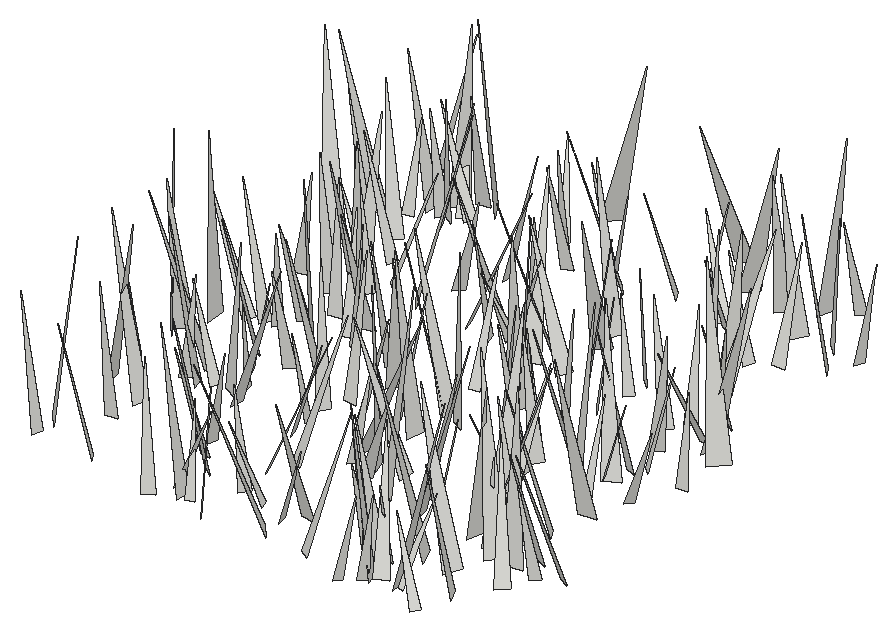
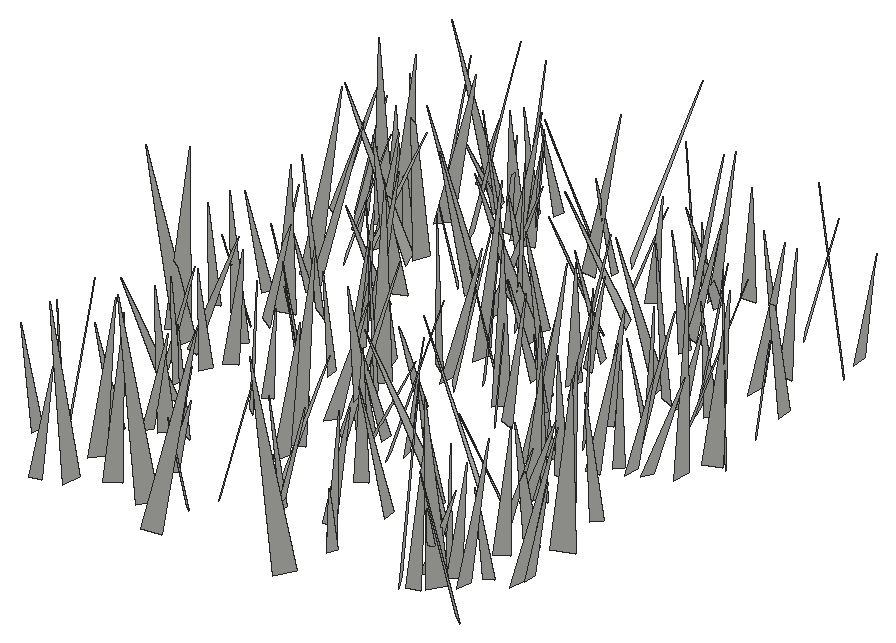
# SketchUp Ruby script. Lengths in inches.
U = 1.inch
M = Sketchup.active_model
def pt(a) = Geom::Point3d.new(a.map { |v| v * U })
def face(e, loops, mat)
  f = e.add_face(loops[0].map { |a| pt(a) })
  loops[1..].each { |l| e.add_face(l.map { |a| pt(a) }).erase! }
  f.material = f.back_material = mat if mat
  f
end
# faces: each face lists its corners as indices into pts; further lists are holes
def faces(e, pts, list, mat = nil) = list.each { |f| face(e, (f[0].is_a?(Array) ? f : [f]).map { |l| l.map { |i| pts[i] } }, mat) }
# xy, xz, yz: faces in a plane at the given z, y or x. An outline is a flat list of corners, or four numbers for a rectangle; further outlines are holes
def ring(l) = l.size == 4 ? [[l[0], l[1]], [l[2], l[1]], [l[2], l[3]], [l[0], l[3]]] : l.each_slice(2).to_a
def flat(e, list, mat, &to3) = list.each { |f| face(e, (f[0].is_a?(Array) ? f : [f]).map { |l| ring(l).map { |u, v| to3.(u, v) } }, mat) }
def xy(e, z, list, mat = nil) = flat(e, list, mat) { |x, y| [x, y, z] }
def xz(e, y, list, mat = nil) = flat(e, list, mat) { |x, z| [x, y, z] }
def yz(e, x, list, mat = nil) = flat(e, list, mat) { |y, z| [x, y, z] }
def lines(e, pts, list) = list.each { |a, b| e.add_line(pt(pts[a]), pt(pts[b])) }
# prism: a flat outline (further loops are holes) pulled along v
def prism(e, loops, v, mat = nil)
  f = face(e, loops, mat); d = Geom::Vector3d.new(v.map { |x| x * U })
  f.pushpull(f.normal.samedirection?(d) ? d.length : -d.length)
end
def box(e, o, s, mat = nil) = prism(e, [[o, [o[0] + s[0], o[1], o[2]], [o[0] + s[0], o[1] + s[1], o[2]], [o[0], o[1] + s[1], o[2]]]], [0, 0, s[2]], mat)
def at(x, y, z, deg = 0) = Geom::Transformation.translation(pt([x, y, z])) * Geom::Transformation.rotation(ORIGIN, Z_AXIS, deg.degrees)
def axes(o, x, y, z) = Geom::Transformation.new([*x, 0, *y, 0, *z, 0, *pt(o).to_a, 1])
def part(name) = M.definitions.add(name)
# library, detail: a bought-in or finely detailed component or shape, given as its bounding box
def library(name, o, s) = part(name).tap { |d| box(d.entities, o, s) }
def detail(e, o, s) = box(e.add_group.entities, o, s)
def put(e, d, t, mat = nil) = e.add_instance(d, t).tap { |i| i.material = mat if mat }
def group(e, t, mat = nil) = e.add_group.tap { |g| g.transformation = t; g.material = mat if mat }.entities
root = M.entities
c1 = part("fur_instance\#9")
p = [[0.8125,0,1.79],[0.67,-0.02,1.48],[0,-0.11,0],[0,0.11,0]]
faces(c1.entities,p,[[0,1,2,3]])
put(root,c1,axes([455.1,295.91,-21.66],[-7.08698,0.49693,1.41438],[0.58095,7.2106,0.37757],[1.38199,-0.48283,7.09434]))
put(root,c1,axes([454.9,294.74,-21.66],[-4.79431,0.50788,0.77321],[0.45097,4.84644,-0.38709],[0.80772,0.30866,4.80557]))
put(root,c1,axes([455.53,290.17,-21.66],[-4.19179,6.94453,1.88873],[7.18228,4.17546,0.58769],[0.45687,-1.92457,8.09026]))
put(root,c1,axes([454.47,272.83,-21.66],[-5.7343,-4.84539,3.53032],[-5.45543,6.24306,-0.29262],[2.4858,2.5238,7.50162]))
put(root,c1,axes([456.32,255.11,-21.66],[-5.31115,0.249,1.00047],[0.14264,5.37711,-0.58108],[1.02108,0.54405,5.28514]))
put(root,c1,axes([455.14,268.49,-21.66],[-2.6203,-2.567,1.06702],[-2.53846,2.80716,0.51965],[1.13325,0.35259,3.63117]))
put(root,c1,axes([455.01,273.69,-21.66],[3.62749,-5.55241,1.8821],[-5.65778,-3.89547,-0.58748],[-1.5366,1.23544,6.60627]))
put(root,c1,axes([455.76,276.27,-21.66],[7.3985,0.06507,3.2704],[0.28828,-8.06925,-0.49163],[-3.25831,-0.56619,7.38244]))
put(root,c1,axes([457.83,277.63,-21.66],[-4.93751,1.50851,0.32737],[1.53378,4.91815,0.47027],[0.1741,-0.54591,5.14135]))
put(root,c1,axes([455.1875,302.65,-21.66],[3.97347,4.57155,1.31094],[4.73936,-3.94824,-0.59665],[-0.39506,-1.38509,6.02757]))
put(root,c1,axes([455.68,264.57,-21.66],[6.8953,0.9557,1.85973],[1.13553,-7.09282,-0.56526],[-1.75571,-0.83402,6.93822]))
put(root,c1,axes([456.08,257.29,-21.66],[5.70767,4.90783,2.44546],[5.23724,-5.92496,-0.33273],[-1.62433,-1.85811,7.52021]))
put(root,c1,axes([458,298.5,-21.66],[-6.22894,0.57755,1.75246],[0.68588,6.45268,0.31131],[1.71297,-0.48351,6.24791]))
put(root,c1,axes([459,278.02,-21.66],[-5.26641,1.25593,0.32091],[1.22212,5.2582,-0.5227],[0.43216,0.43524,5.3888]))
put(root,c1,axes([456.43,285.14,-21.66],[2.66304,-4.00114,1.09323],[-4.14622,-2.60379,0.57024],[-0.11461,1.22768,4.77239]))
put(root,c1,axes([457.17,296.62,-21.66],[-1.25475,3.57203,1.31412],[3.70812,1.4592,-0.42579],[0.858,-1.08261,3.76198]))
put(root,c1,axes([459.375,263.19,-21.66],[-7.31689,1.04904,1.18508],[0.99417,7.40794,-0.41938],[1.23147,0.25252,7.3798]))
put(root,c1,axes([459.79,270.36,-21.66],[-6.57116,-2.81105,0.67584],[-2.85659,6.57143,-0.44162],[0.44572,0.67315,7.13352]))
put(root,c1,axes([458.62,293.32,-21.66],[3.00603,-4.02582,3.59921],[-4.80148,-3.87769,-0.32715],[-2.47129,2.63706,5.01362]))
put(root,c1,axes([457.78,290.93,-21.66],[-1.16882,5.10436,1.64073],[5.31118,1.33199,-0.3603],[0.7334,-1.51127,5.22406]))
put(root,c1,axes([459.01,260.28,-21.66],[-0.51846,-5.08764,2.15235],[-5.51728,0.36879,-0.45728],[-0.27624,2.18298,5.0935]))
put(root,c1,axes([460.64,290.46,-21.66],[-4.9286,0.63717,0.02707],[0.62924,4.89286,-0.60144],[0.10377,0.59304,4.93308]))
put(root,c1,axes([459.24,298,-21.66],[-3.39336,2.50243,2.08506],[2.97495,3.60715,0.51243],[1.32637,-1.68843,4.18502]))
put(root,c1,axes([461.21,298.75,-21.66],[-4.19942,1.95994,0.17006],[1.96728,4.18576,0.33862],[0.01038,-0.37878,4.62189]))
put(root,c1,axes([460.84,267.94,-21.66],[-6.09908,-2.25868,1.59557],[-2.41433,6.23322,-0.4051],[1.3485,0.94419,6.49124]))
put(root,c1,axes([460.5,298.71,-21.66],[-2.92778,3.00983,0.00711],[2.98882,2.90849,-0.48849],[0.35507,0.33555,4.17041]))
put(root,c1,axes([459.98,284.14,-21.66],[1.65081,-5.08845,2.41171],[-5.51574,-1.96719,-0.37505],[-1.13372,2.16141,5.33637]))
put(root,c1,axes([459.32,299.91,-21.66],[6.01123,-4.10409,2.83515],[-4.50522,-6.3728,0.32708],[-2.14119,1.8869,7.27128]))
put(root,c1,axes([459.875,297.85,-21.66],[-2.18081,-4.36379,1.96245],[-4.63729,2.45895,0.31456],[1.17875,1.60022,4.86823]))
put(root,c1,axes([459.56,268.11,-21.66],[2.82184,-3.33686,1.43593],[-3.57868,-2.86589,0.37288],[-0.62414,1.34588,4.35412]))
put(root,c1,axes([461.29,274.18,-21.66],[-3.14093,-4.54056,1.19879],[-4.68857,3.11384,-0.49041],[0.26658,1.26749,5.49924]))
put(root,c1,axes([461.63,254.82,-21.66],[-4.56615,-2.82263,0.99228],[-2.92894,4.58662,-0.43101],[0.61084,0.89289,5.35081]))
put(root,c1,axes([460.02,278.14,-21.66],[3.44775,-2.42349,1.09947],[-2.43313,-3.5995,-0.30427],[-1.07797,0.37336,4.2033]))
put(root,c1,axes([462.16,286.18,-21.66],[-3.83694,1.86592,0.39498],[1.90547,3.78872,0.61201],[0.08273,-0.72368,4.22246]))
put(root,c1,axes([461.96,268.53,-21.66],[-3.54918,2.04608,0.76374],[2.14815,3.53344,0.51649],[0.39398,-0.83357,4.06404]))
put(root,c1,axes([460.53,301.09,-21.66],[1.15457,-5.41906,0.82486],[-5.48032,-1.12384,0.28761],[0.11275,0.86626,5.53322]))
put(root,c1,axes([461.09,279.78,-21.66],[1.69834,-4.62751,0.65795],[-4.61755,-1.76962,-0.52709],[-0.72459,0.43091,4.90106]))
put(root,c1,axes([460.12,296.76,-21.66],[5.04239,2.3615,1.06864],[2.46365,-5.09289,-0.37039],[-0.80566,-0.79378,5.55564]))
put(root,c1,axes([461.84,300.97,-21.66],[-6.4664,-4.252,2.80304],[-4.40658,6.94256,0.3657],[2.55316,1.21333,7.73047]))
put(root,c1,axes([462.0625,285.68,-21.66],[-4.31803,3.62073,2.04082],[3.93255,4.51165,0.31626],[1.34522,-1.56695,5.62628]))
put(root,c1,axes([461.58,285.18,-21.66],[-0.58668,-6.43534,2.37936],[-6.81319,0.82822,0.56013],[0.80964,2.30643,6.43771]))
put(root,c1,axes([462.41,281.7,-21.66],[-0.09344,5.23116,1.72248],[5.50098,0.0052,0.28262],[-0.26677,-1.725,5.22436]))
put(root,c1,axes([462.75,271.79,-21.66],[3.22488,1.438,0.95498],[1.40641,-3.36208,0.31327],[-1.00092,-0.09099,3.51704]))
put(root,c1,axes([464.18,276.92,-21.66],[-5.53367,-3.1899,2.46645],[-3.58117,5.81278,-0.51687],[1.85312,1.70777,6.3663]))
put(root,c1,axes([462.77,287.78,-21.66],[2.99625,3.60782,0.19235],[3.59342,-3.00177,0.328],[-0.37513,0.06212,4.67828]))
put(root,c1,axes([463.48,268.34,-21.66],[-2.04646,-5.42862,2.85461],[-5.95901,2.47232,0.42963],[1.45222,2.49488,5.78561]))
put(root,c1,axes([464.09,269.58,-21.66],[-3.40135,-0.48301,1.73948],[-0.24917,3.80046,0.56808],[1.78802,-0.38922,3.38818]))
put(root,c1,axes([464.97,279.91,-21.66],[-0.50295,4.78104,0.71911],[4.81704,0.43358,0.48636],[-0.41423,-0.76294,4.78276]))
put(root,c1,axes([464.6,273.77,-21.66],[2.46831,-3.73303,1.12427],[-3.72872,-2.64901,-0.60947],[-1.13849,0.58247,4.43358]))
put(root,c1,axes([464.51,282.29,-21.66],[-1.5232,-7.73744,1.34983],[-7.81047,1.63722,0.57115],[0.82858,1.20901,7.86523]))
put(root,c1,axes([465.52,281.71,-21.66],[0.67121,-5.58126,0.90748],[-5.6399,-0.72653,-0.2969],[-0.40679,0.86382,5.61363]))
put(root,c1,axes([466.34,278.82,-21.66],[2.39277,4.07076,1.54907],[4.21231,-2.6123,0.35825],[-1.10775,-1.14055,4.7083]))
put(root,c1,axes([464.87,267.32,-21.66],[6.15775,0.09619,0.89999],[0.03195,-6.20791,0.44493],[-0.90455,0.43558,6.14241]))
put(root,c1,axes([465.71,286.82,-21.66],[6.07013,4.91373,1.22638],[4.90353,-6.18107,0.495],[-1.26656,-0.38061,7.79399]))
put(root,c1,axes([467.77,260.11,-21.66],[-1.24841,-4.57565,0.91997],[-4.66472,1.19209,-0.401],[-0.15278,0.99186,4.72592]))
put(root,c1,axes([468.14,253.0625,-21.66],[-1.55203,4.86816,1.43833],[5.0761,1.479,0.47157],[-0.03172,-1.51332,5.08777]))
put(root,c1,axes([468.5,300.44,-21.66],[-2.98771,2.56269,0.00271],[2.54357,2.96592,-0.47684],[0.31249,0.36018,3.90722]))
put(root,c1,axes([467.01,261.82,-21.66],[4.35751,-1.25814,0.68683],[-1.21703,-4.4086,-0.35441],[-0.75729,-0.15444,4.52164]))
put(root,c1,axes([466.91,290.32,-21.66],[3.70766,-2.56946,0.56874],[-2.62102,-3.69364,0.39947],[-0.23628,0.65362,4.49325]))
put(root,c1,axes([469.375,271.88,-21.66],[-6.2182,-2.45212,1.53392],[-2.39925,6.40419,0.51167],[1.61537,0.0727,6.66461]))
put(root,c1,axes([469.31,258.39,-21.66],[-3.91198,-5.41617,1.52932],[-5.50053,4.07361,0.35664],[1.19076,1.02376,6.67167]))
put(root,c1,axes([470.28,254.41,-21.66],[-6.61174,-0.50833,1.66504],[-0.62205,6.79727,-0.39495],[1.62598,0.53342,6.61948]))
put(root,c1,axes([470.26,270.46,-21.66],[-5.1029,2.41175,1.4356],[2.37658,5.2976,-0.4521],[1.4931,-0.1897,5.62599]))
put(root,c1,axes([468.61,293.75,-21.66],[5.20805,0.62891,1.21236],[0.54515,-5.33937,0.42794],[-1.25226,0.29119,5.2284]))
put(root,c1,axes([470.33,278.13,-21.66],[-1.33118,-5.02308,1.66852],[-5.29255,1.28443,-0.35575],[0.06525,1.70478,5.18429]))
put(root,c1,axes([469.64,299.1,-21.66],[-0.67343,-4.75938,1.30258],[-4.88536,0.82798,0.49956],[0.69398,1.21023,4.78075]))
put(root,c1,axes([470.8,268.25,-21.66],[-0.62514,-3.66803,1.11265],[-3.82799,0.53943,-0.37244],[-0.19721,1.15663,3.70223]))
put(root,c1,axes([471.07,278.57,-21.66],[-3.53133,-2.30027,1.49102],[-2.55807,3.63918,-0.44418],[0.98523,1.20406,4.19097]))
put(root,c1,axes([471.07,254.19,-21.66],[-0.33834,3.74046,0.53618],[3.75079,0.26714,0.50319],[-0.45836,-0.57497,3.72187]))
put(root,c1,axes([469.18,255.26,-21.66],[3.86855,-0.79855,0.19754],[-0.81455,-3.85123,0.38332],[-0.11496,0.41562,3.93147]))
put(root,c1,axes([471.09,297.55,-21.66],[0.8668,-4.44855,1.11397],[-4.54098,-0.99091,-0.42373],[-0.6404,1.00517,4.51236]))
put(root,c1,axes([471.12,272.55,-21.66],[0.82489,5.68831,1.342],[5.81529,-0.93413,0.38496],[-0.58339,-1.2684,5.73491]))
put(root,c1,axes([469.12,305.09,-21.66],[6.86151,-4.43995,0.81428],[-4.49635,-6.85344,0.51929],[-0.39875,0.87961,8.15621]))
put(root,c1,axes([470.72,266.56,-21.66],[4.18181,1.0835,0.53294],[1.13424,-4.18373,-0.39425],[-0.41412,-0.51766,4.30187]))
put(root,c1,axes([474.02,287.125,-21.66],[-6.24569,-2.79636,0.92417],[-2.76847,6.31368,0.39421],[1.00464,0.01396,6.83176]))
put(root,c1,axes([470.65,286.79,-21.66],[5.67742,2.27779,0.25934],[2.25803,-5.67581,0.41845],[-0.39608,0.29237,6.10297]))
put(root,c1,axes([473.16,286.06,-21.66],[-4.36965,-1.59831,1.51111],[-1.58231,4.61869,0.30967],[1.52785,0.21216,4.64247]))
put(root,c1,axes([473.3125,257.71,-21.66],[-3.08367,2.72536,1.78242],[3.08151,3.23588,0.38343],[1.05304,-1.48834,4.09751]))
put(root,c1,axes([472.31,276.29,-21.66],[4.37125,-4.19897,0.80164],[-4.19734,-4.43318,-0.33332],[-0.81017,0.31203,6.05212]))
put(root,c1,axes([472.9,253.22,-21.66],[4.36466,2.86173,1.95624],[3.18404,-4.55325,-0.44325],[-1.3705,-1.46462,5.20032]))
put(root,c1,axes([472.875,271.71,-21.66],[4.10361,0.18993,0.89205],[0.09258,-4.17709,0.46346],[-0.90734,0.43277,4.08178]))
put(root,c1,axes([473.18,291.27,-21.66],[1.74282,-4.6233,0.69197],[-4.67126,-1.6936,0.44965],[0.18179,0.80496,4.92038]))
put(root,c1,axes([475.42,297.72,-21.66],[-4.70558,-0.80345,0.83315],[-0.88013,4.74917,-0.39105],[0.7517,0.53106,4.75763]))
put(root,c1,axes([476.07,297.59,-21.66],[-5.08924,-4.37631,0.84531],[-4.44671,5.07308,-0.50754],[0.30556,0.93743,6.69289]))
put(root,c1,axes([473.67,263.17,-21.66],[2.91229,5.1803,0.24137],[5.15397,-2.92189,0.52374],[-0.57474,0.04729,5.91968]))
put(root,c1,axes([472.66,261.24,-21.66],[5.42276,2.60915,0.23648],[2.58182,-5.41452,0.53583],[-0.44475,0.3811,5.9939]))
put(root,c1,axes([475.55,257.0625,-21.66],[-3.47043,-1.20582,0.35373],[-1.16309,3.47557,0.43669],[0.47575,-0.29913,3.64791]))
put(root,c1,axes([476.55,285.76,-21.66],[-3.57731,-0.93265,0.01118],[-0.92223,3.54345,0.51048],[0.1395,-0.49118,3.66148]))
put(root,c1,axes([475.42,274.39,-21.66],[3.95748,1.9361,2.48086],[2.44941,-4.39763,-0.47534],[-1.97573,-1.57388,4.37997]))
put(root,c1,axes([477.72,275.67,-21.66],[-6.93734,1.12272,0.61983],[1.08478,6.95591,-0.45824],[0.68406,0.3553,7.01265]))
put(root,c1,axes([476.79,276.17,-21.66],[-5.18557,-4.32883,1.54546],[-4.49087,5.26797,-0.31293],[0.97941,1.23577,6.74766]))
put(root,c1,axes([475.15,273.24,-21.66],[3.56693,3.32971,1.1246],[3.34181,-3.70943,0.38354],[-1.08812,-0.47732,4.86445]))
put(root,c1,axes([475.125,297.73,-21.66],[4.21688,0.53755,0.91963],[0.65776,-4.26755,-0.52159],[-0.83787,-0.64478,4.21888]))
put(root,c1,axes([478.08,254.125,-21.66],[-5.65228,-5.31186,0.60473],[-5.29476,5.68375,0.43618],[0.73959,0.09466,7.74428]))
put(root,c1,axes([476.91,279.5625,-21.66],[0.03105,4.61747,0.04613],[4.59439,-0.03553,0.46309],[-0.46341,-0.04278,4.59429]))
put(root,c1,axes([475.76,285.19,-21.66],[4.29201,-0.29938,0.77765],[-0.39482,-4.32378,0.51456],[-0.73381,0.57535,4.27156]))
put(root,c1,axes([477.57,285.27,-21.66],[-1.40207,7.22786,1.13046],[7.31414,1.36087,0.37039],[-0.15287,-1.17973,7.35327]))
put(root,c1,axes([477.78,271.74,-21.66],[-7.15931,0.95304,2.49675],[1.12982,7.54938,0.35801],[2.42189,-0.70454,7.21359]))
put(root,c1,axes([478.25,287.04,-21.66],[-4.17901,-5.88434,0.7845],[-5.89024,4.22956,0.34775],[0.73891,0.43633,7.20893]))
put(root,c1,axes([476.8,265.77,-21.66],[3.29573,-2.04708,1.27302],[-2.29025,-3.33183,0.57152],[-0.75223,1.17531,3.83742]))
put(root,c1,axes([478.625,266.47,-21.66],[-6.27895,-2.5321,2.5957],[-2.9165,6.61067,-0.60625],[2.15482,1.56906,6.74309]))
put(root,c1,axes([479.9,292.08,-21.66],[-6.40273,2.01611,1.14645],[1.98655,6.50456,-0.34415],[1.19695,-0.01086,6.70383]))
put(root,c1,axes([480.54,285.39,-21.66],[-5.38349,2.8617,0.60302],[2.91403,5.35589,0.59819],[0.24775,-0.81245,6.06741]))
put(root,c1,axes([479.19,274.78,-21.66],[3.04497,5.63186,2.55497],[5.93211,-3.46487,0.56775],[-1.7481,-1.94792,6.3771]))
put(root,c1,axes([476.43,267.45,-21.66],[6.73911,-0.51973,0.37006],[-0.5475,-6.72675,0.52311],[-0.32757,0.55072,6.73884]))
put(root,c1,axes([481.02,266.62,-21.66],[-6.42244,0.41118,0.57395],[0.45958,6.42194,0.54196],[0.53597,-0.57954,6.41273]))
put(root,c1,axes([479.72,299.37,-21.66],[-3.92886,-2.51502,0.86647],[-2.44083,4.02285,0.60923],[1.05758,-0.05874,4.62495]))
put(root,c1,axes([478.06,256.09,-21.66],[3.62066,0.28745,0.41277],[0.34104,-3.60783,-0.479],[-0.36973,-0.51296,3.60033]))
put(root,c1,axes([479.46,257.36,-21.66],[-0.57876,-6.04691,0.53315],[-6.05695,0.61084,0.35302],[0.40347,0.49606,6.06428]))
put(root,c1,axes([478.83,264.7,-21.66],[3.52002,-2.83902,0.00242],[-2.82378,-3.50072,0.47096],[0.29379,0.3681,4.49764]))
put(root,c1,axes([480.45,306.32,-21.66],[1.9178,-7.47283,0.23219],[-7.45531,-1.92947,-0.52008],[-0.56157,0.09505,7.69744]))
put(root,c1,axes([480.29,280.63,-21.66],[6.26613,3.81902,2.82967],[4.24719,-6.60086,-0.4964],[-2.13385,-1.92357,7.3214]))
put(root,c1,axes([480.49,302.07,-21.66],[2.6007,2.51832,0.88377],[2.64819,-2.58836,-0.41733],[-0.33183,-0.9193,3.59603]))
put(root,c1,axes([480.32,289.98,-21.66],[4.1786,-6.03386,0.40804],[-6.0035,-4.19846,-0.60465],[-0.72937,-0.01047,7.31455]))
put(root,c1,axes([481.125,279.0625,-21.66],[6.49174,-3.69034,2.54193],[-3.75607,-6.92147,-0.45599],[-2.44375,0.83512,7.45341]))
put(root,c1,axes([481.62,263.65,-21.66],[4.31651,6.80061,2.35568],[7.01576,-4.58865,0.3914],[-1.60519,-1.76799,8.04533]))
put(root,c1,axes([482.29,276.13,-21.66],[4.52412,1.43506,1.852],[1.32361,-4.8885,0.5546],[-1.93323,0.01133,4.71375]))
put(root,c1,axes([482.82,285.21,-21.66],[4.79862,3.05458,1.6678],[3.017,-5.06719,0.60002],[-1.73486,-0.36311,5.65661]))
put(root,c1,axes([482.41,253.2,-21.66],[3.35621,4.76804,0.53975],[4.75729,-3.3924,0.38655],[-0.62744,-0.21695,5.81798]))
put(root,c1,axes([484.73,298.5,-21.66],[-3.18645,2.79123,0.05753],[2.78151,3.16651,0.42911],[-0.23972,-0.36053,4.21429]))
put(root,c1,axes([485.49,275.99,-21.66],[-3.44021,1.49763,0.22694],[1.46636,3.43395,-0.43273],[0.37973,0.30751,3.72702]))
put(root,c1,axes([484.77,280.17,-21.66],[4.11345,0.18865,1.81103],[0.00918,-4.47631,0.44541],[-1.8208,0.4036,4.09361]))
put(root,c1,axes([485.69,255.96,-21.66],[-3.35833,-3.2337,1.73378],[-3.57177,3.41915,-0.54142],[0.83981,1.61055,4.63056]))
put(root,c1,axes([485.76,275.54,-21.66],[-4.49863,-0.46507,1.40367],[-0.60193,4.68178,-0.37796],[1.35065,0.53749,4.50678]))
put(root,c1,axes([485.54,297.73,-21.66],[-1.12897,-3.54048,0.33773],[-3.515,1.16474,0.46018],[0.54205,0.17891,3.68752]))
put(root,c1,axes([485.36,256.84,-21.66],[2.55514,-3.36467,0.69917],[-3.31318,-2.64324,-0.61213],[-0.91251,0.1757,4.18031]))
put(root,c1,axes([486.12,285.82,-21.66],[1.74245,-3.02379,2.07472],[-3.3962,-2.19711,-0.34987],[-1.38332,1.58534,3.47232]))
put(root,c1,axes([483.3125,303.18,-21.66],[6.15872,-4.73604,0.69713],[-4.78091,-6.14284,0.50431],[-0.2428,0.82545,7.75278]))
put(root,c1,axes([484.47,264.65,-21.66],[5.61379,-0.0924,1.25595],[-0.17391,-5.73971,0.3551],[-1.24727,0.38445,5.60331]))
put(root,c1,axes([486.77,256.42,-21.66],[-5.40914,1.11965,1.3835],[1.23539,5.5484,0.3398],[1.28121,-0.62292,5.51334]))
put(root,c1,axes([485.84,288.09,-21.66],[-2.86919,-3.90872,1.79506],[-4.01549,3.2075,0.56601],[1.54149,1.08002,4.8156]))
put(root,c1,axes([485.77,264.41,-21.66],[-2.4957,-1.61977,2.11338],[-2.18018,2.90599,-0.34732],[1.52869,1.50005,2.95492]))
put(root,c1,axes([485.67,282.7,-21.66],[3.79573,2.84609,1.46317],[3.05532,-3.89817,-0.34352],[-0.95191,-1.16307,4.73179]))
put(root,c1,axes([487.05,274.07,-21.66],[-4.02078,2.93374,1.78068],[3.22926,4.16274,0.43339],[1.1617,-1.41743,4.95839]))
put(root,c1,axes([487.45,272.06,-21.66],[5.36084,-0.19835,3.29768],[0.06393,-6.27827,-0.48156],[-3.30302,-0.44345,5.34285]))
put(root,c1,axes([485.42,262.89,-21.66],[6.99973,1.86447,1.44835],[1.77883,-7.14461,0.6004],[-1.55233,0.22015,7.21886]))
put(root,c1,axes([487.3125,293.83,-21.66],[1.36793,4.62634,1.5435],[4.80198,-1.5578,0.41343],[-0.85231,-1.35162,4.8066]))
put(root,c1,axes([486.66,251.76,-21.66],[3.38987,-1.12165,1.00676],[-1.27426,-3.45624,0.43994],[-0.80492,0.7478,3.54341]))
put(root,c1,axes([488.33,253.51,-21.66],[5.38161,2.47127,3.67462],[2.66712,-6.4254,0.41515],[-3.53503,-1.08568,5.90733]))
put(root,c1,axes([487.1,302.375,-21.66],[3.86717,-5.0611,1.49434],[-5.13106,-4.03908,-0.40116],[-1.23289,0.93486,6.35679]))
put(root,c1,axes([489.05,253.78,-21.66],[-1.93628,5.55,0.46539],[5.55779,1.89356,0.54185],[-0.36056,-0.61659,5.85304]))
put(root,c1,axes([487.84,256.1875,-21.66],[-0.65259,-3.58567,0.77528],[-3.62638,0.74954,0.41412],[0.55447,0.682,3.62097]))
put(root,c1,axes([489.5,258.33,-21.66],[-7.3935,-3.44968,1.78048],[-3.41196,7.60131,0.55924],[1.85173,0.23234,8.13949]))
put(root,c1,axes([488.4,268.17,-21.66],[-2.23719,7.0676,1.63885],[7.20712,2.3619,-0.34736],[0.83319,-1.45336,7.40509]))
put(root,c1,axes([488.31,269.63,-21.66],[-0.0626,5.05917,0.30688],[5.04763,0.09003,-0.45456],[0.45914,-0.29998,5.03909]))
put(root,c1,axes([488.04,252.85,-21.66],[2.26375,-3.28304,0.92587],[-3.40814,-2.22313,0.4499],[-0.14199,1.01955,3.96238]))
put(root,c1,axes([489.94,294.82,-21.66],[-4.10178,1.61092,0.95507],[1.70987,4.15942,0.32775],[0.76391,-0.66031,4.39457]))
put(root,c1,axes([488.66,294.2,-21.66],[3.55242,-4.27149,1.91187],[-4.60398,-3.6203,0.46613],[-0.83917,1.77997,5.53606]))
put(root,c1,axes([490.32,300.14,-21.66],[-5.43342,3.18473,2.47254],[3.60205,5.6984,0.57576],[1.81141,-1.77869,6.27161]))
put(root,c1,axes([489.57,304.0625,-21.66],[6.98669,-0.82296,2.45735],[-1.02769,-7.36659,0.45485],[-2.37901,0.76535,7.02027]))
put(root,c1,axes([492.32,257.86,-21.66],[-6.29408,3.56033,1.19684],[3.6784,6.31519,0.55815],[0.76008,-1.07993,7.20971]))
put(root,c1,axes([491.29,283.6,-21.66],[-3.65531,3.57205,1.42816],[3.77376,3.712,0.37448],[0.74692,-1.27356,5.09712]))
put(root,c1,axes([491.04,273.75,-21.66],[3.25616,5.95918,2.11371],[6.15078,-3.5363,0.49462],[-1.46542,-1.60155,6.77272]))
put(root,c1,axes([490.75,253.61,-21.66],[0.42201,3.83383,0.13948],[3.79822,-0.3978,-0.55775],[0.53966,-0.19825,3.81644]))
put(root,c1,axes([490.32,262.95,-21.66],[6.63287,-1.89646,1.66739],[-1.83678,-6.83922,-0.47211],[-1.73291,-0.0097,6.88248]))
put(root,c1,axes([492.88,272.33,-21.66],[-3.74984,-6.28849,1.24601],[-6.40364,3.74219,-0.38514],[0.30173,1.26879,7.3115]))
put(root,c1,axes([491.78,305.43,-21.66],[1.41164,-4.04262,0.99191],[-4.10193,-1.52908,-0.39425],[-0.70768,0.79907,4.26381]))
put(root,c1,axes([491.24,290.3,-21.66],[0.40052,6.46259,0.29319],[6.45769,-0.38185,-0.40475],[0.38629,-0.31712,6.46233]))
put(root,c1,axes([493.66,265.01,-21.66],[-3.87501,-4.05549,0.17386],[-4.05477,3.85598,-0.42797],[-0.18982,0.42113,5.59281]))
put(root,c1,axes([490.58,253.78,-21.66],[7.58691,1.58366,1.76713],[1.48707,-7.78642,0.59349],[-1.84915,0.23586,7.72768]))
put(root,c1,axes([492.99,275.28,-21.66],[-2.95923,6.17255,1.7602],[6.41346,2.92118,0.53848],[0.25723,-1.82266,6.82403]))
put(root,c1,axes([492.26,285.31,-21.66],[-3.32764,3.062,1.30373],[3.08153,3.53122,-0.42827],[1.25687,-0.55083,4.50173]))
put(root,c1,axes([491.84,295.83,-21.66],[-0.34341,4.80516,0.97397],[4.88667,0.41477,-0.32328],[0.39826,-0.94579,4.80656]))
put(root,c1,axes([493.12,277.26,-21.66],[-2.87551,-4.98025,1.4124],[-5.17006,2.84441,-0.49611],[0.26119,1.47404,5.72934]))
put(root,c1,axes([493.68,263.61,-21.66],[-5.54027,1.19429,0.93196],[1.15956,5.61711,-0.30487],[0.97482,0.10593,5.65933]))
put(root,c1,axes([493.75,251.74,-21.66],[-2.71204,2.5664,0.21286],[2.56651,2.66825,0.52947],[-0.21147,-0.53003,3.69611]))
put(root,c1,axes([493.58,261.26,-21.66],[-6.05615,5.17907,2.30301],[5.46239,6.23254,0.34836],[1.51293,-1.77094,7.96105]))
put(root,c1,axes([492.16,262.1,-21.66],[2.05705,-3.40779,1.21765],[-3.60141,-2.06493,0.30505],[-0.3543,1.20424,3.9688]))
put(root,c1,axes([494.51,266.53,-21.66],[-5.00716,-3.11226,0.75462],[-3.18598,4.98296,-0.58898],[0.32424,0.90067,5.86608]))
put(root,c1,axes([493.23,272.01,-21.66],[0.25291,3.93977,0.05992],[3.89833,-0.25892,0.57035],[-0.57304,-0.02262,3.90646]))
put(root,c1,axes([490.86,263.67,-21.66],[6.96857,2.87265,0.80723],[2.85827,-7.01507,0.2896],[-0.85676,-0.03815,7.53188]))
put(root,c1,axes([492.21,275.43,-21.66],[3.27913,1.40298,0.59687],[1.4938,-3.23974,-0.59158],[-0.30522,-0.78299,3.51725]))
put(root,c1,axes([492.57,288.23,-21.66],[3.92592,-0.41216,0.89749],[-0.2951,-4.00034,-0.54626],[-0.94248,-0.46433,3.90952]))
put(root,c1,axes([493.3,300.1875,-21.66],[-3.24328,-4.06122,2.56752],[-4.33534,3.80899,0.54855],[2.07134,1.61325,5.16831]))
put(root,c1,axes([492.73,280.72,-21.66],[3.51068,-4.45404,1.06123],[-4.56743,-3.50052,0.41776],[-0.32136,1.09429,5.65587]))
put(root,c1,axes([494.74,286.7,-21.66],[-2.89308,-3.13599,0.85003],[-3.23039,2.89836,-0.3018],[0.34876,0.83187,4.25597]))
put(root,c1,axes([494.59,283.88,-21.66],[-0.95692,-4.60949,0.0097],[-4.59629,0.95343,-0.35816],[-0.34872,0.08227,4.69412]))
put(root,c1,axes([494.96,297.55,-21.66],[-5.04486,-3.51647,1.75014],[-3.733,5.17856,-0.35556],[1.22196,1.30239,6.1392]))
put(root,c1,axes([494.55,255.09,-21.66],[4.53456,1.85789,3.16607],[2.55783,-5.20835,-0.60709],[-2.63311,-1.85992,4.86266]))
put(root,c1,axes([493.96,278.09,-21.66],[2.60004,3.22909,0.64132],[3.22546,-2.66223,0.32783],[-0.65933,-0.2899,4.13277]))
put(root,c1,axes([494.83,270.13,-21.66],[0.47812,-7.3143,1.47747],[-7.45136,-0.54714,-0.29732],[-0.39895,1.45332,7.32388]))
put(root,c1,axes([496.67,258.07,-21.66],[-4.29612,3.71614,0.38084],[3.69784,4.31285,-0.36964],[0.52979,0.03157,5.66831]))
put(root,c1,axes([495.29,260.97,-21.66],[1.282,-6.99581,3.06835],[-7.6361,-1.26107,0.31524],[-0.21483,3.07701,7.10532]))
put(root,c1,axes([496.43,262.84,-21.66],[-1.84979,-4.95748,0.73449],[-4.97918,1.90688,0.3307],[0.56907,0.57009,5.281]))
put(root,c1,axes([497.51,281.93,-21.66],[-5.36752,5.77658,2.45123],[6.12108,5.53013,0.37117],[1.38195,-2.05828,7.87664]))
put(root,c1,axes([496.09,299.84,-21.66],[4.13039,-0.87619,1.21239],[-0.99071,-4.26996,0.28929],[-1.12075,0.54542,4.21238]))
put(root,c1,axes([495.9375,273.59,-21.66],[3.40491,-1.73217,0.1961],[-1.74293,-3.39081,0.31125],[-0.03288,0.3664,3.80749]))
put(root,c1,axes([497.7,260.61,-21.66],[1.52237,-3.55739,1.37163],[-3.65271,-1.78416,-0.57315],[-1.09275,1.00785,3.82677]))
put(root,c1,axes([495.8,283.17,-21.66],[7.40162,-2.04644,1.37858],[-2.14984,-7.48787,0.42713],[-1.21103,0.78507,7.66743]))
put(root,c1,axes([497.63,277.5,-21.66],[0.95056,-3.70171,1.6828],[-4.06505,-0.90725,0.30052],[-0.09921,1.70654,3.80998]))
put(root,c1,axes([499.51,261.61,-21.66],[-3.13069,-4.74867,0.6646],[-4.79451,3.11096,-0.35688],[0.06511,0.75154,5.67659]))
